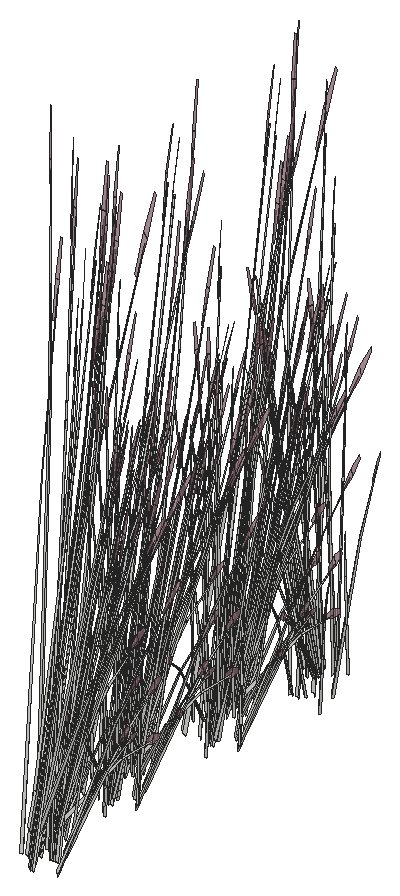
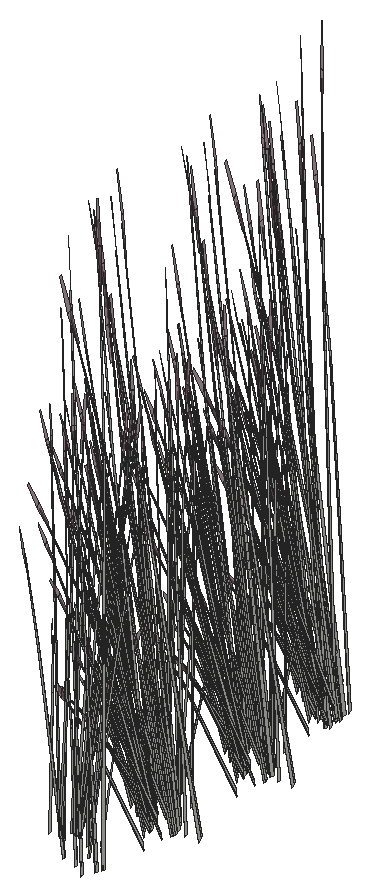
# SketchUp Ruby script. Lengths in inches.
U = 1.inch
M = Sketchup.active_model
def pt(a) = Geom::Point3d.new(a.map { |v| v * U })
def face(e, loops, mat)
  f = e.add_face(loops[0].map { |a| pt(a) })
  loops[1..].each { |l| e.add_face(l.map { |a| pt(a) }).erase! }
  f.material = f.back_material = mat if mat
  f
end
# faces: each face lists its corners as indices into pts; further lists are holes
def faces(e, pts, list, mat = nil) = list.each { |f| face(e, (f[0].is_a?(Array) ? f : [f]).map { |l| l.map { |i| pts[i] } }, mat) }
# xy, xz, yz: faces in a plane at the given z, y or x. An outline is a flat list of corners, or four numbers for a rectangle; further outlines are holes
def ring(l) = l.size == 4 ? [[l[0], l[1]], [l[2], l[1]], [l[2], l[3]], [l[0], l[3]]] : l.each_slice(2).to_a
def flat(e, list, mat, &to3) = list.each { |f| face(e, (f[0].is_a?(Array) ? f : [f]).map { |l| ring(l).map { |u, v| to3.(u, v) } }, mat) }
def xy(e, z, list, mat = nil) = flat(e, list, mat) { |x, y| [x, y, z] }
def xz(e, y, list, mat = nil) = flat(e, list, mat) { |x, z| [x, y, z] }
def yz(e, x, list, mat = nil) = flat(e, list, mat) { |y, z| [x, y, z] }
def lines(e, pts, list) = list.each { |a, b| e.add_line(pt(pts[a]), pt(pts[b])) }
# prism: a flat outline (further loops are holes) pulled along v
def prism(e, loops, v, mat = nil)
  f = face(e, loops, mat); d = Geom::Vector3d.new(v.map { |x| x * U })
  f.pushpull(f.normal.samedirection?(d) ? d.length : -d.length)
end
def box(e, o, s, mat = nil) = prism(e, [[o, [o[0] + s[0], o[1], o[2]], [o[0] + s[0], o[1] + s[1], o[2]], [o[0], o[1] + s[1], o[2]]]], [0, 0, s[2]], mat)
def at(x, y, z, deg = 0) = Geom::Transformation.translation(pt([x, y, z])) * Geom::Transformation.rotation(ORIGIN, Z_AXIS, deg.degrees)
def axes(o, x, y, z) = Geom::Transformation.new([*x, 0, *y, 0, *z, 0, *pt(o).to_a, 1])
def part(name) = M.definitions.add(name)
# library, detail: a bought-in or finely detailed component or shape, given as its bounding box
def library(name, o, s) = part(name).tap { |d| box(d.entities, o, s) }
def detail(e, o, s) = box(e.add_group.entities, o, s)
def put(e, d, t, mat = nil) = e.add_instance(d, t).tap { |i| i.material = mat if mat }
def group(e, t, mat = nil) = e.add_group.tap { |g| g.transformation = t; g.material = mat if mat }.entities
root = M.entities
M.materials.add("LightPink_Translucent").color = [144, 107, 117]
M.materials["LightPink_Translucent"].alpha = 0.75
c1 = part("blade")
p = [[2.15,0.21,22],[0,0.17,0],[0.09,0.45,0],[2.18,0.31,22],[2.29,0.31,22],[0.38,0.45,0],
  [2.48,0.24,33],[2.49,0.24,33],[2.48,0.22,33]]
faces(c1.entities,p,[[0,1,2,3],[4,5,2,3],[6,3,4,7],[8,0,3,6]])
c2 = part("seeds")
p = [[0.3,-0.1,1.38],[-0.01,-0.03,1.59],[-0.01,-0.03,0.03],[0.14,-0.07,-0.07],[0.29,-0.03,3],[0.15,0.01,3.11]]
faces(c2.entities,p,[[0,1,2,3],[1,0,4,5]],"LightPink_Translucent")
c3 = part("blade with seeds")
put(c3.entities,c1,at(0,0,0))
put(c3.entities,c2,axes([2.4,0.25,30.99],[1.5799,-0.05474,1.17369],[-0.12525,1.92788,0.29478],[-0.07173,-0.02425,1.56792]))
put(root,c3,axes([407.81,364.76,-10.61],[-0.02673,-0.08252,1.6421],[0.18538,-0.48271,-0.25086],[0.187,-0.00694,0.2797]))
put(root,c3,axes([405.03,364.2,-9.47],[-0.30722,-0.45622,0.41661],[0.46535,-0.32126,-0.2005],[0.09942,0.05645,1.33761]))
put(root,c3,axes([405.1875,364.23,-9.52],[0.51635,-0.36087,-0.27094],[0.34336,0.5099,-0.46562],[0.1274,0.05178,1.4872]))
put(root,c3,axes([407.24,365.18,-7.78],[0.42502,0.15163,-0.32977],[-0.12396,0.44238,0.42575],[0.17112,-0.04056,0.81462]))
put(root,c3,axes([406.49,363.27,-10.12],[0.47863,0.27177,-0.46235],[-0.28609,0.48733,0],[0.10901,0.0619,1.46668]))
put(root,c3,axes([405.58,364.82,-9.95],[0.57217,0,0],[0,0.56272,0],[0,0,1.66132]))
put(root,c3,axes([406.08,364.64,-8.39],[-0.21212,0.01231,1.59586],[0.14072,-0.53355,0.12904],[0.3023,0.033,0.68222]))
put(root,c3,axes([406.36,363.48,-10.11],[0.12013,0.47362,-0.28847],[-0.47712,0.13449,0.28847],[0.09619,0.05462,1.29413]))
put(root,c3,axes([407.18,365.37,-7.6],[0.18783,0.37061,0.05988],[-0.34252,0.1814,0.47138],[0.15099,-0.03579,0.71878]))
put(root,c3,axes([407.14,365.24,-7.59],[-0.14449,0.4956,0.447],[-0.47502,-0.16947,0.36857],[0.1868,-0.02978,0.92496]))
put(root,c3,axes([405.5,366.07,-9.97],[0.53691,-0.18442,-0.17877],[0.18866,0.53125,0.00007],[0.05927,-0.02038,1.61933]))
put(root,c3,axes([405.79,364.3125,-10.08],[0.53199,0.08911,-0.58063],[-0.11226,0.54969,-0.15239],[0.15876,0.06661,1.28164]))
put(root,c3,axes([408.14,365.27,-9.42],[-0.31598,0.08973,1.06958],[0.14873,-0.37085,0.78586],[0.16763,0.02538,0.23558]))
put(root,c3,axes([407.99,366.84,-7.62],[-0.04624,-0.04758,1.65179],[0.10116,-0.51007,-0.15608],[0.18215,-0.03259,0.29231]))
put(root,c3,axes([405.51,364.49,-9.94],[0.30722,0.45622,-0.41661],[-0.46535,0.32126,0.2005],[0.09942,0.05645,1.33761]))
put(root,c3,axes([407.59,366.42,-8.34],[-0.09788,-0.45691,-0.03251],[0.46264,-0.10504,-0.14742],[0.09661,0.02897,0.48626]))
put(root,c3,axes([406.39,366.4,-7.3125],[0.02738,-0.55277,-0.11324],[0.51847,0.01511,-0.62851],[0.19968,0.0384,0.95501]))
put(root,c3,axes([406.87,364.93,-9.69],[0,-0.54355,0.46235],[0.57217,0,0],[0,0.1238,1.46668]))
put(root,c3,axes([405.78,364.76,-9.5625],[0.47648,-0.15851,0.13483],[0.16686,0.45265,-0.38503],[0,0.09962,1.18024]))
put(root,c3,axes([406.3125,366.1875,-7.3],[-0.29098,-0.34031,0.32977],[0.33226,-0.32215,-0.42575],[0.16881,0.04902,0.81462]))
put(root,c3,axes([407.55,365.87,-9.59],[-0.12317,-0.13368,1.33163],[0.16025,-0.44223,-0.28638],[0.24919,0.05991,0.56934]))
put(root,c3,axes([406.84,366.07,-7.61],[0.10971,-0.00919,1.62908],[0.30091,-0.42228,-0.25764],[0.19514,0.05574,0.13065]))
put(root,c3,axes([406.42,366.14,-7.36],[0.51122,0.01309,-0.66157],[-0.03434,0.5511,0.07984],[0.21658,0.05816,0.93586]))
put(root,c3,axes([407.25,365.02,-9.79],[0.63949,0,0],[0,0.60749,-0.48057],[0,0.13836,1.52448]))
put(root,c3,axes([405.61,364.8,-9.52],[0.57594,0.25935,-0.27094],[-0.27732,0.5474,-0.46562],[0.0181,0.1344,1.4872]))
put(root,c3,axes([406.73,366.36,-7.78],[0.29098,0.34031,-0.32977],[-0.33226,0.32215,0.42575],[0.16881,0.04902,0.81462]))
put(root,c3,axes([406.86,365.42,-10.11],[-0.35699,0.33913,-0.28847],[-0.35699,-0.33913,0.28847],[0,0.10923,1.29413]))
put(root,c3,axes([406.58,366.49,-7.6],[-0.02575,0.41332,0.05988],[-0.38885,-0.01133,0.47138],[0.14895,0.04325,0.71878]))
put(root,c3,axes([406.61,366.36,-7.59],[-0.37709,0.35815,0.447],[-0.32522,-0.38035,0.36857],[0.17692,0.06607,0.92496]))
put(root,c3,axes([405.41,366.78,-7.3],[-0.07899,-0.43781,0.32977],[0.45153,-0.11561,-0.42575],[0.12128,0.12546,0.81462]))
put(root,c3,axes([407.11,365.43,-10.12],[0,0.54355,-0.46235],[-0.57217,0,0],[0,0.1238,1.46668]))
put(root,c3,axes([405.68,365.49,-8.39],[-0.18996,-0.09365,1.59586],[0.39312,-0.39287,0.12904],[0.24502,0.17723,0.68222]))
put(root,c3,axes([405.72,364.26,-7.83],[-0.44191,-0.28242,1.28769],[0.46662,-0.43971,0.5556],[0.14258,0.26499,1.24467]))
put(root,c3,axes([406.38,366.56,-9.42],[-0.28795,-0.15629,1.06958],[0.37181,-0.1588,0.78586],[0.10029,0.13452,0.23558]))
put(root,c3,axes([405.37,367,-7.3125],[0.30474,-0.46525,-0.11324],[0.44133,0.26804,-0.62851],[0.15341,0.13145,0.95501]))
put(root,c3,axes([404.97,367.39,-7.62],[0.00151,-0.06581,1.65179],[0.43826,-0.29033,-0.15608],[0.15223,0.10363,0.29231]))
put(root,c3,axes([406.46,367.14,-10.61],[0.03726,-0.07847,1.6421],[0.46909,-0.23111,-0.25086],[0.14221,0.11962,0.2797]))
put(root,c3,axes([405.84,365.36,-10.05],[0.18752,0.49766,-0.6445],[-0.54017,0.17923,-0.16915],[0.02073,0.16852,1.42262]))
put(root,c3,axes([405.73,366.77,-7.64],[0.50465,-0.12921,-0.47583],[0.08828,0.48932,-0.36857],[0.13555,0.14022,0.91046]))
put(root,c3,axes([405.29,373.04,-7.61],[-0.00494,-0.10818,1.62908],[-0.41695,-0.31265,-0.25764],[0.06446,-0.18952,0.13065]))
put(root,c3,axes([403.875,373.57,-8.39],[-0.09522,0.18683,1.59586],[-0.39947,-0.38663,0.12904],[0.18021,-0.24097,0.68222]))
put(root,c3,axes([406.43,367.27,-9.52],[-0.32795,-0.01705,0.97832],[0.21658,-0.36206,0.54015],[0.12956,0.12863,0.76741]))
put(root,c3,axes([405.48,367.17,-7.6],[-0.23243,0.34529,0.05988],[-0.331,-0.20103,0.47138],[0.10701,0.1107,0.71878]))
put(root,c3,axes([405.58,367.08,-7.59],[-0.50866,0.12474,0.447],[-0.08828,-0.48932,0.36857],[0.11963,0.14421,0.92496]))
put(root,c3,axes([405.36,366.39,-9.59],[0.00902,-0.18018,1.33163],[0.43127,-0.20126,-0.28638],[0.13313,0.21566,0.56934]))
put(root,c3,axes([404.9,366.04,-8.39],[-0.1169,-0.17452,1.59586],[0.54019,-0.14692,0.12904],[0.12209,0.27397,0.68222]))
put(root,c3,axes([405.17,373.35,-10.61],[-0.07655,-0.04282,1.6421],[-0.19662,-0.47839,-0.25086],[0.13264,-0.12982,0.2797]))
put(root,c3,axes([404.73,373.63,-7.59],[0.36417,0.37086,0.447],[-0.38674,0.31985,0.36857],[0.06718,-0.174,0.92496]))
put(root,c3,axes([404.87,373.67,-7.6],[0.42027,0.02533,0.05988],[-0.01152,0.38243,0.47138],[0.04398,-0.14649,0.71878]))
put(root,c3,axes([405.16,374.7,-7.36],[0.26714,-0.42887,-0.66157],[0.46811,0.30479,0.07984],[0.1595,-0.15539,0.93586]))
put(root,c3,axes([405.15,374.5,-7.64],[-0.13138,-0.49631,-0.47583],[0.49754,-0.08682,-0.36857],[0.14258,-0.13331,0.91046]))
put(root,c3,axes([405.39,374.85,-7.3125],[-0.47307,-0.29971,-0.11324],[0.27254,-0.43404,-0.62851],[0.13365,-0.15087,0.95501]))
put(root,c3,axes([405.55,374.3,-9.59],[-0.1827,-0.0161,1.33163],[-0.18717,-0.43188,-0.28638],[0.22444,-0.12218,0.56934]))
put(root,c3,axes([406.55,374.72,-7.62],[-0.0668,-0.00413,1.65179],[-0.27738,-0.44233,-0.15608],[0.11139,-0.14544,0.29231]))
put(root,c3,axes([403.28,374.48,-10.08],[0.34446,-0.40855,-0.58063],[0.42791,0.37046,-0.15239],[0.13803,-0.10191,1.28164]))
put(root,c3,axes([405.76,373.51,-9.42],[-0.17034,0.27669,1.06958],[-0.14642,-0.37174,0.78586],[0.14069,-0.09315,0.23558]))
put(root,c3,axes([405.52,374.55,-7.78],[0.44516,-0.07768,-0.32977],[0.11755,0.44407,0.42575],[0.12757,-0.11927,0.81462]))
put(root,c3,axes([405.16,374.8125,-7.3],[-0.44516,0.07768,0.32977],[-0.11755,-0.44407,-0.42575],[0.12757,-0.11927,0.81462]))
put(root,c3,axes([405.56,374.74,-7.6],[0.35109,0.22859,0.05988],[-0.2044,0.32553,0.47138],[0.11256,-0.10524,0.71878]))
put(root,c3,axes([405.46,374.65,-7.59],[0.12683,0.50025,0.447],[-0.49754,0.08682,0.36857],[0.14663,-0.11765,0.92496]))
put(root,c3,axes([406.8,375.25,-7.61],[0.07097,-0.08279,1.62908],[-0.09083,-0.50786,-0.25764],[0.17806,-0.09629,0.13065]))
put(root,c3,axes([405.4,376.02,-7.3125],[-0.25732,-0.49218,-0.11324],[0.45669,-0.24187,-0.62851],[0.19245,-0.06494,0.95501]))
put(root,c3,axes([405.38,375.6,-7.64],[0.13855,-0.49442,-0.47583],[0.47502,0.16947,-0.36857],[0.19125,-0.04534,0.91046]))
put(root,c3,axes([404.63,373.59,-9.79],[0.31974,-0.54466,0],[0.53494,0.30375,-0.48057],[0.12184,0.06918,1.52448]))
put(root,c3,axes([405.89,375.74,-10.15],[-0.32938,0.06523,1.31842],[-0.05243,-0.51922,0.07547],[0.2307,-0.07859,0.75023]))
put(root,c3,axes([406.49,375.28,-9.89],[-0.31706,-0.34757,-0.06041],[0.34725,-0.31847,-0.27392],[0.09839,-0.02242,0.90349]))
put(root,c3,axes([405.29,375.78,-7.36],[0.44939,-0.24006,-0.66157],[0.25044,0.49415,0.07984],[0.21713,-0.05613,0.93586]))
put(root,c3,axes([405.23,375.875,-7.3],[-0.42502,-0.15163,0.32977],[0.12396,-0.44238,-0.42575],[0.17112,-0.04056,0.81462]))
put(root,c3,axes([402.32,374.55,-10.52],[-0.50338,0.21762,1.20058],[-0.16022,-0.62439,0.4665],[0.30911,0.01039,1.36553]))
put(root,c3,axes([406.25,375.4,-10.61],[-0.02673,-0.08252,1.6421],[0.18538,-0.48271,-0.25086],[0.187,-0.00694,0.2797]))
put(root,c3,axes([403.62,374.875,-9.52],[0.51635,-0.36087,-0.27094],[0.34336,0.5099,-0.46562],[0.1274,0.05178,1.4872]))
put(root,c3,axes([405.67,375.82,-7.78],[0.42502,0.15163,-0.32977],[-0.12396,0.44238,0.42575],[0.17112,-0.04056,0.81462]))
put(root,c3,axes([404.92,373.91,-10.12],[0.47863,0.27177,-0.46235],[-0.28609,0.48733,0],[0.10901,0.0619,1.46668]))
put(root,c3,axes([404.52,375.28,-8.39],[-0.21212,0.01231,1.59586],[0.14072,-0.53355,0.12904],[0.3023,0.033,0.68222]))
put(root,c3,axes([404.79,374.12,-10.11],[0.12013,0.47362,-0.28847],[-0.47712,0.13449,0.28847],[0.09619,0.05462,1.29413]))
put(root,c3,axes([405.61,376.01,-7.6],[0.18783,0.37061,0.05988],[-0.34252,0.1814,0.47138],[0.15099,-0.03579,0.71878]))
put(root,c3,axes([405.57,375.88,-7.59],[-0.14449,0.4956,0.447],[-0.47502,-0.16947,0.36857],[0.1868,-0.02978,0.92496]))
put(root,c3,axes([404.22,374.95,-10.08],[0.53199,0.08911,-0.58063],[-0.11226,0.54969,-0.15239],[0.15876,0.06661,1.28164]))
put(root,c3,axes([406.57,375.91,-9.42],[-0.31598,0.08973,1.06958],[0.14873,-0.37085,0.78586],[0.16763,0.02538,0.23558]))
put(root,c3,axes([406.43,377.48,-7.62],[-0.04624,-0.04758,1.65179],[0.10116,-0.51007,-0.15608],[0.18215,-0.03259,0.29231]))
put(root,c3,axes([406.03,377.06,-8.34],[-0.09788,-0.45691,-0.03251],[0.46264,-0.10504,-0.14742],[0.09661,0.02897,0.48626]))
put(root,c3,axes([404.83,377.04,-7.3125],[0.02738,-0.55277,-0.11324],[0.51847,0.01511,-0.62851],[0.19968,0.0384,0.95501]))
put(root,c3,axes([404.75,376.83,-7.3],[-0.29098,-0.34031,0.32977],[0.33226,-0.32215,-0.42575],[0.16881,0.04902,0.81462]))
put(root,c3,axes([405.98,376.51,-9.59],[-0.12317,-0.13368,1.33163],[0.16025,-0.44223,-0.28638],[0.24919,0.05991,0.56934]))
put(root,c3,axes([405.28,376.71,-7.61],[0.10971,-0.00919,1.62908],[0.30091,-0.42228,-0.25764],[0.19514,0.05574,0.13065]))
put(root,c3,axes([404.85,376.78,-7.36],[0.51122,0.01309,-0.66157],[-0.03434,0.5511,0.07984],[0.21658,0.05816,0.93586]))
put(root,c3,axes([405.6875,375.66,-9.79],[0.63949,0,0],[0,0.60749,-0.48057],[0,0.13836,1.52448]))
put(root,c3,axes([405.16,377.01,-7.78],[0.29098,0.34031,-0.32977],[-0.33226,0.32215,0.42575],[0.16881,0.04902,0.81462]))
put(root,c3,axes([405.01,377.14,-7.6],[-0.02575,0.41332,0.05988],[-0.38885,-0.01133,0.47138],[0.14895,0.04325,0.71878]))
put(root,c3,axes([405.05,377,-7.59],[-0.37709,0.35815,0.447],[-0.32522,-0.38035,0.36857],[0.17692,0.06607,0.92496]))
put(root,c3,axes([404.11,376.13,-8.39],[-0.18996,-0.09365,1.59586],[0.39312,-0.39287,0.12904],[0.24502,0.17723,0.68222]))
put(root,c3,axes([404.82,377.2,-9.42],[-0.28795,-0.15629,1.06958],[0.37181,-0.1588,0.78586],[0.10029,0.13452,0.23558]))
put(root,c3,axes([403.81,377.65,-7.3125],[0.30474,-0.46525,-0.11324],[0.44133,0.26804,-0.62851],[0.15341,0.13145,0.95501]))
put(root,c3,axes([403.41,378.03,-7.62],[0.00151,-0.06581,1.65179],[0.43826,-0.29033,-0.15608],[0.15223,0.10363,0.29231]))
put(root,c3,axes([404.9,377.78,-10.61],[0.03726,-0.07847,1.6421],[0.46909,-0.23111,-0.25086],[0.14221,0.11962,0.2797]))
put(root,c3,axes([404.17,377.42,-7.64],[0.50465,-0.12921,-0.47583],[0.08828,0.48932,-0.36857],[0.13555,0.14022,0.91046]))
put(root,c3,axes([404.86,377.91,-9.52],[-0.32795,-0.01705,0.97832],[0.21658,-0.36206,0.54015],[0.12956,0.12863,0.76741]))
put(root,c3,axes([405.57,383.9,-7.61],[-0.00494,-0.10818,1.62908],[-0.41695,-0.31265,-0.25764],[0.06446,-0.18952,0.13065]))
put(root,c3,axes([404.15,384.43,-8.39],[-0.09522,0.18683,1.59586],[-0.39947,-0.38663,0.12904],[0.18021,-0.24097,0.68222]))
put(root,c3,axes([403.79,377.03,-9.59],[0.00902,-0.18018,1.33163],[0.43127,-0.20126,-0.28638],[0.13313,0.21566,0.56934]))
put(root,c3,axes([405.02,384.38,-7.78],[0.34603,-0.28618,-0.32977],[0.32756,0.32677,0.42575],[0.04984,-0.16603,0.81462]))
put(root,c3,axes([405.45,384.21,-10.61],[-0.07655,-0.04282,1.6421],[-0.19662,-0.47839,-0.25086],[0.13264,-0.12982,0.2797]))
put(root,c3,axes([405.01,384.49,-7.59],[0.36417,0.37086,0.447],[-0.38674,0.31985,0.36857],[0.06718,-0.174,0.92496]))
put(root,c3,axes([405.15,384.53,-7.6],[0.42027,0.02533,0.05988],[-0.01152,0.38243,0.47138],[0.04398,-0.14649,0.71878]))
put(root,c3,axes([405.44,385.56,-7.36],[0.26714,-0.42887,-0.66157],[0.46811,0.30479,0.07984],[0.1595,-0.15539,0.93586]))
put(root,c3,axes([405.43,385.36,-7.64],[-0.13138,-0.49631,-0.47583],[0.49754,-0.08682,-0.36857],[0.14258,-0.13331,0.91046]))
put(root,c3,axes([405.67,385.71,-7.3125],[-0.47307,-0.29971,-0.11324],[0.27254,-0.43404,-0.62851],[0.13365,-0.15087,0.95501]))
put(root,c3,axes([405.83,385.16,-9.59],[-0.1827,-0.0161,1.33163],[-0.18717,-0.43188,-0.28638],[0.22444,-0.12218,0.56934]))
put(root,c3,axes([406.83,385.58,-7.62],[-0.0668,-0.00413,1.65179],[-0.27738,-0.44233,-0.15608],[0.11139,-0.14544,0.29231]))
put(root,c3,axes([403.56,385.34,-10.08],[0.34446,-0.40855,-0.58063],[0.42791,0.37046,-0.15239],[0.13803,-0.10191,1.28164]))
put(root,c3,axes([406.04,384.37,-9.42],[-0.17034,0.27669,1.06958],[-0.14642,-0.37174,0.78586],[0.14069,-0.09315,0.23558]))
put(root,c3,axes([405.8,385.41,-7.78],[0.44516,-0.07768,-0.32977],[0.11755,0.44407,0.42575],[0.12757,-0.11927,0.81462]))
put(root,c3,axes([405.44,385.67,-7.3],[-0.44516,0.07768,0.32977],[-0.11755,-0.44407,-0.42575],[0.12757,-0.11927,0.81462]))
put(root,c3,axes([405.84,385.6,-7.6],[0.35109,0.22859,0.05988],[-0.2044,0.32553,0.47138],[0.11256,-0.10524,0.71878]))
put(root,c3,axes([405.74,385.5,-7.59],[0.12683,0.50025,0.447],[-0.49754,0.08682,0.36857],[0.14663,-0.11765,0.92496]))
put(root,c3,axes([407.08,386.11,-7.61],[0.07097,-0.08279,1.62908],[-0.09083,-0.50786,-0.25764],[0.17806,-0.09629,0.13065]))
put(root,c3,axes([405.69,386.88,-7.3125],[-0.25732,-0.49218,-0.11324],[0.45669,-0.24187,-0.62851],[0.19245,-0.06494,0.95501]))
put(root,c3,axes([405.66,386.46,-7.64],[0.13855,-0.49442,-0.47583],[0.47502,0.16947,-0.36857],[0.19125,-0.04534,0.91046]))
put(root,c3,axes([404.91,384.45,-9.79],[0.31974,-0.54466,0],[0.53494,0.30375,-0.48057],[0.12184,0.06918,1.52448]))
put(root,c3,axes([406.17,386.6,-10.15],[-0.32938,0.06523,1.31842],[-0.05243,-0.51922,0.07547],[0.2307,-0.07859,0.75023]))
put(root,c3,axes([406.77,386.14,-9.89],[-0.31706,-0.34757,-0.06041],[0.34725,-0.31847,-0.27392],[0.09839,-0.02242,0.90349]))
put(root,c3,axes([405.57,386.64,-7.36],[0.44939,-0.24006,-0.66157],[0.25044,0.49415,0.07984],[0.21713,-0.05613,0.93586]))
put(root,c3,axes([405.51,386.73,-7.3],[-0.42502,-0.15163,0.32977],[0.12396,-0.44238,-0.42575],[0.17112,-0.04056,0.81462]))
put(root,c3,axes([402.6,385.41,-10.52],[-0.50338,0.21762,1.20058],[-0.16022,-0.62439,0.4665],[0.30911,0.01039,1.36553]))
put(root,c3,axes([406.53,386.26,-10.61],[-0.02673,-0.08252,1.6421],[0.18538,-0.48271,-0.25086],[0.187,-0.00694,0.2797]))
put(root,c3,axes([403.9,385.73,-9.52],[0.51635,-0.36087,-0.27094],[0.34336,0.5099,-0.46562],[0.1274,0.05178,1.4872]))
put(root,c3,axes([405.95,386.68,-7.78],[0.42502,0.15163,-0.32977],[-0.12396,0.44238,0.42575],[0.17112,-0.04056,0.81462]))
put(root,c3,axes([405.2,384.77,-10.12],[0.47863,0.27177,-0.46235],[-0.28609,0.48733,0],[0.10901,0.0619,1.46668]))
put(root,c3,axes([404.8,386.14,-8.39],[-0.21212,0.01231,1.59586],[0.14072,-0.53355,0.12904],[0.3023,0.033,0.68222]))
put(root,c3,axes([405.07,384.98,-10.11],[0.12013,0.47362,-0.28847],[-0.47712,0.13449,0.28847],[0.09619,0.05462,1.29413]))
put(root,c3,axes([405.89,386.87,-7.6],[0.18783,0.37061,0.05988],[-0.34252,0.1814,0.47138],[0.15099,-0.03579,0.71878]))
put(root,c3,axes([405.86,386.74,-7.59],[-0.14449,0.4956,0.447],[-0.47502,-0.16947,0.36857],[0.1868,-0.02978,0.92496]))
put(root,c3,axes([404.5,385.8125,-10.08],[0.53199,0.08911,-0.58063],[-0.11226,0.54969,-0.15239],[0.15876,0.06661,1.28164]))
put(root,c3,axes([406.86,386.77,-9.42],[-0.31598,0.08973,1.06958],[0.14873,-0.37085,0.78586],[0.16763,0.02538,0.23558]))
put(root,c3,axes([406.71,388.34,-7.62],[-0.04624,-0.04758,1.65179],[0.10116,-0.51007,-0.15608],[0.18215,-0.03259,0.29231]))
put(root,c3,axes([404.23,385.99,-9.94],[0.30722,0.45622,-0.41661],[-0.46535,0.32126,0.2005],[0.09942,0.05645,1.33761]))
put(root,c3,axes([406.31,387.92,-8.34],[-0.09788,-0.45691,-0.03251],[0.46264,-0.10504,-0.14742],[0.09661,0.02897,0.48626]))
put(root,c3,axes([405.11,387.9,-7.3125],[0.02738,-0.55277,-0.11324],[0.51847,0.01511,-0.62851],[0.19968,0.0384,0.95501]))
put(root,c3,axes([405.03,387.6875,-7.3],[-0.29098,-0.34031,0.32977],[0.33226,-0.32215,-0.42575],[0.16881,0.04902,0.81462]))
put(root,c3,axes([406.26,387.37,-9.59],[-0.12317,-0.13368,1.33163],[0.16025,-0.44223,-0.28638],[0.24919,0.05991,0.56934]))
put(root,c3,axes([405.56,387.57,-7.61],[0.10971,-0.00919,1.62908],[0.30091,-0.42228,-0.25764],[0.19514,0.05574,0.13065]))
put(root,c3,axes([405.13,387.64,-7.36],[0.51122,0.01309,-0.66157],[-0.03434,0.5511,0.07984],[0.21658,0.05816,0.93586]))
put(root,c3,axes([405.97,386.52,-9.79],[0.63949,0,0],[0,0.60749,-0.48057],[0,0.13836,1.52448]))
put(root,c3,axes([405.44,387.87,-7.78],[0.29098,0.34031,-0.32977],[-0.33226,0.32215,0.42575],[0.16881,0.04902,0.81462]))
put(root,c3,axes([406.74,393.55,-9.59],[-0.14537,0.11002,1.33163],[-0.43536,-0.19256,-0.28638],[0.0807,-0.23948,0.56934]))
put(root,c3,axes([405.29,388,-7.6],[-0.02575,0.41332,0.05988],[-0.38885,-0.01133,0.47138],[0.14895,0.04325,0.71878]))
put(root,c3,axes([405.33,387.86,-7.59],[-0.37709,0.35815,0.447],[-0.32522,-0.38035,0.36857],[0.17692,0.06607,0.92496]))
put(root,c3,axes([407.09,394.37,-7.36],[0.01331,-0.50278,-0.66157],[0.56035,0.03377,0.07984],[0.05914,-0.213,0.93586]))
put(root,c3,axes([404.13,388.28,-7.3],[-0.07899,-0.43781,0.32977],[0.45153,-0.11561,-0.42575],[0.12128,0.12546,0.81462]))
put(root,c3,axes([407.87,393.58,-7.61],[-0.00494,-0.10818,1.62908],[-0.41695,-0.31265,-0.25764],[0.06446,-0.18952,0.13065]))
put(root,c3,axes([406.46,394.11,-8.39],[-0.09522,0.18683,1.59586],[-0.39947,-0.38663,0.12904],[0.18021,-0.24097,0.68222]))
put(root,c3,axes([407.76,393.19,-7.62],[-0.05194,0.04152,1.65179],[-0.50886,-0.14007,-0.15608],[-0.01842,-0.18118,0.29231]))
put(root,c3,axes([404.39,386.99,-8.39],[-0.18996,-0.09365,1.59586],[0.39312,-0.39287,0.12904],[0.24502,0.17723,0.68222]))
put(root,c3,axes([404.43,385.76,-7.83],[-0.44191,-0.28242,1.28769],[0.46662,-0.43971,0.5556],[0.14258,0.26499,1.24467]))
put(root,c3,axes([406.2,392.68,-9.42],[0.06561,0.31695,1.06958],[-0.36394,-0.17555,0.78586],[0.03916,-0.16229,0.23558]))
put(root,c3,axes([405.1,388.06,-9.42],[-0.28795,-0.15629,1.06958],[0.37181,-0.1588,0.78586],[0.10029,0.13452,0.23558]))
put(root,c3,axes([406.98,394.2,-7.64],[-0.3661,-0.36521,-0.47583],[0.38674,-0.31985,-0.36857],[0.0557,-0.18556,0.91046]))
put(root,c3,axes([404.09,388.51,-7.3125],[0.30474,-0.46525,-0.11324],[0.44133,0.26804,-0.62851],[0.15341,0.13145,0.95501]))
put(root,c3,axes([403.6875,388.89,-7.62],[0.00151,-0.06581,1.65179],[0.43826,-0.29033,-0.15608],[0.15223,0.10363,0.29231]))
put(root,c3,axes([406.18,393.66,-7.59],[0.50393,0.1421,0.447],[-0.17232,0.46717,0.36857],[-0.03028,-0.18372,0.92496]))
put(root,c3,axes([405.18,388.64,-10.61],[0.03726,-0.07847,1.6421],[0.46909,-0.23111,-0.25086],[0.14221,0.11962,0.2797]))
put(root,c3,axes([407.36,394.39,-7.3125],[-0.56206,-0.02693,-0.11324],[0.01536,-0.50991,-0.62851],[0.03904,-0.19638,0.95501]))
put(root,c3,axes([407.32,394.07,-7.78],[0.34603,-0.28618,-0.32977],[0.32756,0.32677,0.42575],[0.04984,-0.16603,0.81462]))
put(root,c3,axes([404.45,388.27,-7.64],[0.50465,-0.12921,-0.47583],[0.08828,0.48932,-0.36857],[0.13555,0.14022,0.91046]))
put(root,c3,axes([406.31,393.62,-7.6],[0.37684,-0.18473,0.05988],[0.18445,0.33686,0.47138],[-0.03639,-0.14849,0.71878]))
put(root,c3,axes([405.14,388.77,-9.52],[-0.32795,-0.01705,0.97832],[0.21658,-0.36206,0.54015],[0.12956,0.12863,0.76741]))
put(root,c3,axes([407.75,393.89,-10.61],[-0.07655,-0.04282,1.6421],[-0.19662,-0.47839,-0.25086],[0.13264,-0.12982,0.2797]))
put(root,c3,axes([404.07,387.89,-9.59],[0.00902,-0.18018,1.33163],[0.43127,-0.20126,-0.28638],[0.13313,0.21566,0.56934]))
put(root,c3,axes([407.32,394.18,-7.59],[0.36417,0.37086,0.447],[-0.38674,0.31985,0.36857],[0.06718,-0.174,0.92496]))
put(root,c3,axes([407.45,394.21,-7.6],[0.42027,0.02533,0.05988],[-0.01152,0.38243,0.47138],[0.04398,-0.14649,0.71878]))
put(root,c3,axes([407.14,394.47,-7.3],[-0.34603,0.28618,0.32977],[-0.32756,-0.32677,-0.42575],[0.04984,-0.16603,0.81462]))
put(root,c3,axes([407.75,395.24,-7.36],[0.26714,-0.42887,-0.66157],[0.46811,0.30479,0.07984],[0.1595,-0.15539,0.93586]))
put(root,c3,axes([404.86,393.99,-9.79],[-0.31974,-0.54466,0],[0.53494,-0.30375,-0.48057],[0.12184,-0.06918,1.52448]))
put(root,c3,axes([407.74,395.04,-7.64],[-0.13138,-0.49631,-0.47583],[0.49754,-0.08682,-0.36857],[0.14258,-0.13331,0.91046]))
put(root,c3,axes([407.97,395.4,-7.3125],[-0.47307,-0.29971,-0.11324],[0.27254,-0.43404,-0.62851],[0.13365,-0.15087,0.95501]))
put(root,c3,axes([405.3,393.91,-10.12],[0.47863,-0.27177,-0.46235],[0.28609,0.48733,0],[0.10901,-0.0619,1.46668]))
put(root,c3,axes([408.14,394.85,-9.59],[-0.1827,-0.0161,1.33163],[-0.18717,-0.43188,-0.28638],[0.22444,-0.12218,0.56934]))
put(root,c3,axes([409.14,395.27,-7.62],[-0.0668,-0.00413,1.65179],[-0.27738,-0.44233,-0.15608],[0.11139,-0.14544,0.29231]))
put(root,c3,axes([405.86,395.02,-10.08],[0.34446,-0.40855,-0.58063],[0.42791,0.37046,-0.15239],[0.13803,-0.10191,1.28164]))
